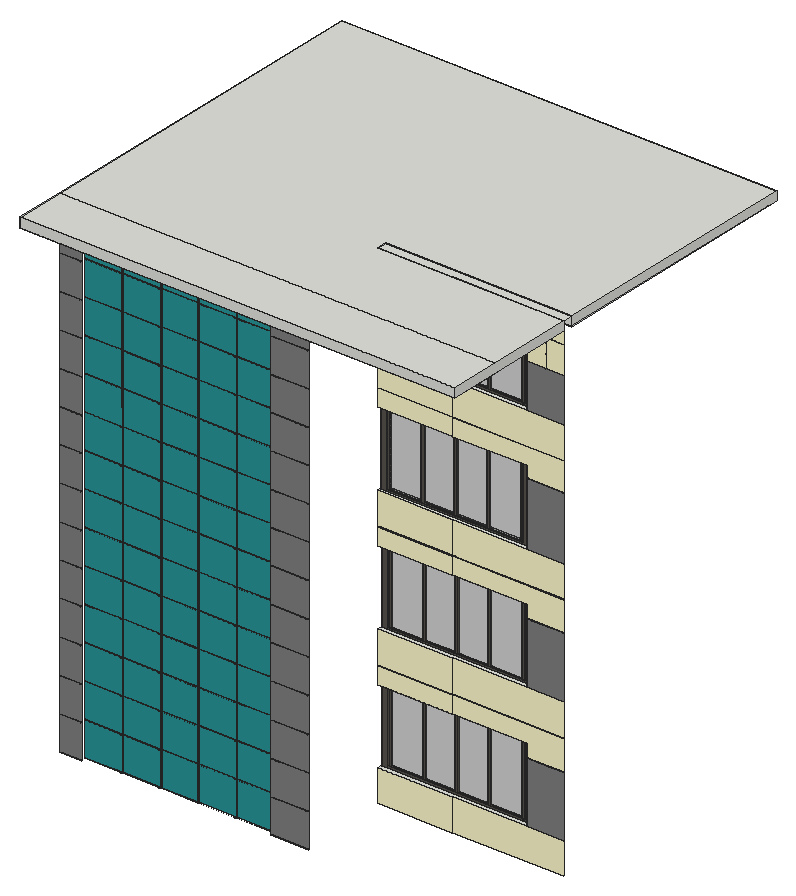
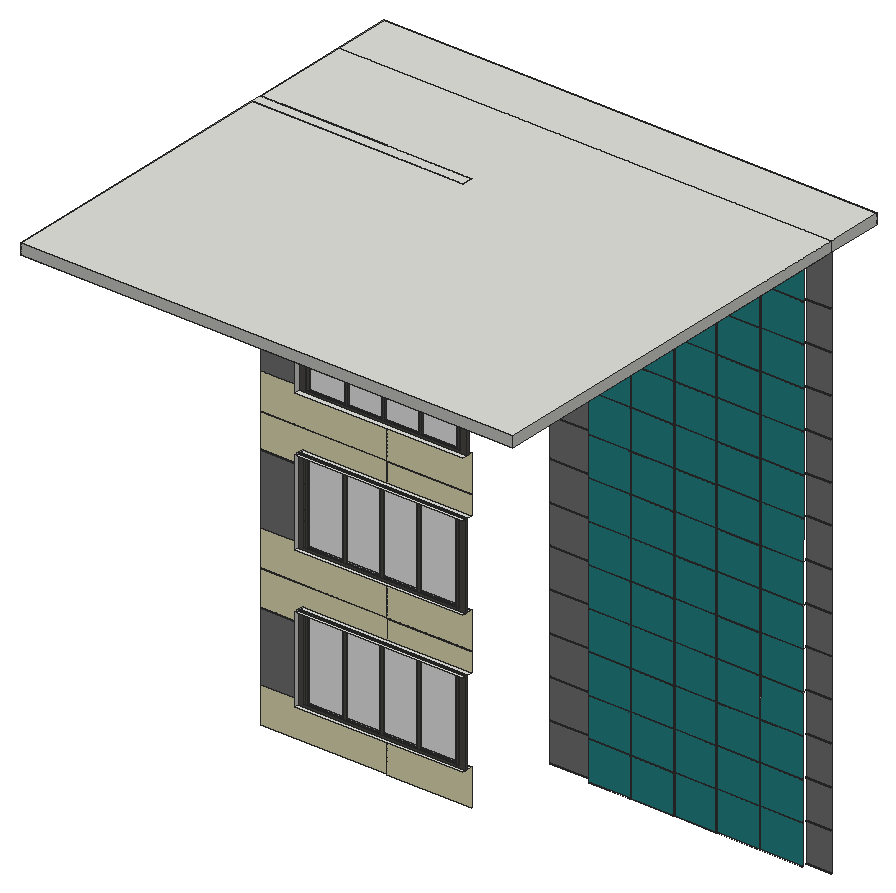
# SketchUp Ruby script. Lengths in inches.
U = 1.inch
M = Sketchup.active_model
def pt(a) = Geom::Point3d.new(a.map { |v| v * U })
def face(e, loops, mat)
  f = e.add_face(loops[0].map { |a| pt(a) })
  loops[1..].each { |l| e.add_face(l.map { |a| pt(a) }).erase! }
  f.material = f.back_material = mat if mat
  f
end
# faces: each face lists its corners as indices into pts; further lists are holes
def faces(e, pts, list, mat = nil) = list.each { |f| face(e, (f[0].is_a?(Array) ? f : [f]).map { |l| l.map { |i| pts[i] } }, mat) }
# xy, xz, yz: faces in a plane at the given z, y or x. An outline is a flat list of corners, or four numbers for a rectangle; further outlines are holes
def ring(l) = l.size == 4 ? [[l[0], l[1]], [l[2], l[1]], [l[2], l[3]], [l[0], l[3]]] : l.each_slice(2).to_a
def flat(e, list, mat, &to3) = list.each { |f| face(e, (f[0].is_a?(Array) ? f : [f]).map { |l| ring(l).map { |u, v| to3.(u, v) } }, mat) }
def xy(e, z, list, mat = nil) = flat(e, list, mat) { |x, y| [x, y, z] }
def xz(e, y, list, mat = nil) = flat(e, list, mat) { |x, z| [x, y, z] }
def yz(e, x, list, mat = nil) = flat(e, list, mat) { |y, z| [x, y, z] }
def lines(e, pts, list) = list.each { |a, b| e.add_line(pt(pts[a]), pt(pts[b])) }
# prism: a flat outline (further loops are holes) pulled along v
def prism(e, loops, v, mat = nil)
  f = face(e, loops, mat); d = Geom::Vector3d.new(v.map { |x| x * U })
  f.pushpull(f.normal.samedirection?(d) ? d.length : -d.length)
end
def box(e, o, s, mat = nil) = prism(e, [[o, [o[0] + s[0], o[1], o[2]], [o[0] + s[0], o[1] + s[1], o[2]], [o[0], o[1] + s[1], o[2]]]], [0, 0, s[2]], mat)
def at(x, y, z, deg = 0) = Geom::Transformation.translation(pt([x, y, z])) * Geom::Transformation.rotation(ORIGIN, Z_AXIS, deg.degrees)
def axes(o, x, y, z) = Geom::Transformation.new([*x, 0, *y, 0, *z, 0, *pt(o).to_a, 1])
def part(name) = M.definitions.add(name)
# library, detail: a bought-in or finely detailed component or shape, given as its bounding box
def library(name, o, s) = part(name).tap { |d| box(d.entities, o, s) }
def detail(e, o, s) = box(e.add_group.entities, o, s)
def put(e, d, t, mat = nil) = e.add_instance(d, t).tap { |i| i.material = mat if mat }
def group(e, t, mat = nil) = e.add_group.tap { |g| g.transformation = t; g.material = mat if mat }.entities
root = M.entities
M.materials.add("Aluminum_Anodized_DarkGray").color = [87, 83, 78]
M.materials.add("Glass_Coated_Black").color = [65, 65, 65]
M.materials["Glass_Coated_Black"].alpha = 0.42
M.materials.add("[0050_LemonChiffon]").color = [255, 250, 205]
M.materials.add("[0081_CadetBlue]").color = [40, 149, 153]
M.materials.add("[0133_Gray]").color = [128, 128, 128]
M.materials.add("[0137_Black]").color = [0, 0, 0]
c1 = part("Group\#2")
xy(c1.entities,0,[[0,0,54,3]],"Aluminum_Anodized_DarkGray")
xy(c1.entities,2,[[2.25,0,51.75,1],[2.25,2,51.75,3]],"Aluminum_Anodized_DarkGray")
xy(c1.entities,3,[[3.375,1,14.625,1.5],[15.75,1,26.4375,1.5],[27.5625,1,38.25,1.5],[39.375,1,50.625,1.5],[3.375,1.5,14.625,2],
  [15.75,1.5,26.4375,2],[27.5625,1.5,38.25,2],[39.375,1.5,50.625,2]],"Aluminum_Anodized_DarkGray")
xy(c1.entities,99,[[3.375,1,14.625,1.5],[15.75,1,26.4375,1.5],[26.4375,1,27.5625,2],[27.5625,1,38.25,1.5],[38.25,1,39.375,2],
  [39.375,1,50.625,1.5],[3.375,1.5,14.625,2],[15.75,1.5,26.4375,2],[27.5625,1.5,38.25,2],[39.375,1.5,50.625,2]],"Aluminum_Anodized_DarkGray")
xy(c1.entities,100,[[2.25,0,51.75,1],[2.25,2,51.75,3]],"Aluminum_Anodized_DarkGray")
xy(c1.entities,102,[[0,0,54,3]],"Aluminum_Anodized_DarkGray")
xz(c1.entities,0,[[[0,0,54,102],[2.25,2,51.75,100]]],"Aluminum_Anodized_DarkGray")
xz(c1.entities,1,[[[2.25,2,51.75,100],[39.375,3,50.625,99],[3.375,3,14.625,99],[27.5625,3,38.25,99],[15.75,3,26.4375,99]]],"Aluminum_Anodized_DarkGray")
xz(c1.entities,1.5,[[3.375,3,14.625,99],[15.75,3,27,99],[27.5625,3,38.8125,99],[39.375,3,50.625,99]],"Glass_Coated_Black")
xz(c1.entities,2,[[[2.25,2,51.75,100],[39.375,3,50.625,99],[3.375,3,14.625,99],[27.5625,3,38.25,99],[15.75,3,26.4375,99]]],"Aluminum_Anodized_DarkGray")
xz(c1.entities,3,[[[0,0,54,102],[2.25,2,51.75,100]]],"Aluminum_Anodized_DarkGray")
yz(c1.entities,0,[[0,0,3,102]],"Aluminum_Anodized_DarkGray")
yz(c1.entities,2.25,[[0,2,1,100],[2,2,3,100]],"Aluminum_Anodized_DarkGray")
yz(c1.entities,3.375,[[1,3,1.5,99],[1.5,3,2,99]],"Aluminum_Anodized_DarkGray")
yz(c1.entities,14.625,[[1,3,1.5,99],[1.5,3,2,99]],"Aluminum_Anodized_DarkGray")
yz(c1.entities,15.75,[[1,3,1.5,99],[1.5,3,2,99]],"Aluminum_Anodized_DarkGray")
yz(c1.entities,26.4375,[[1,3,2,99]],"Aluminum_Anodized_DarkGray")
yz(c1.entities,27.5625,[[1,3,1.5,99],[1.5,3,2,99]],"Aluminum_Anodized_DarkGray")
yz(c1.entities,38.25,[[1,3,2,99]],"Aluminum_Anodized_DarkGray")
yz(c1.entities,39.375,[[1,3,1.5,99],[1.5,3,2,99]],"Aluminum_Anodized_DarkGray")
yz(c1.entities,50.625,[[1,3,1.5,99],[1.5,3,2,99]],"Aluminum_Anodized_DarkGray")
yz(c1.entities,51.75,[[0,2,1,100],[2,2,3,100]],"Aluminum_Anodized_DarkGray")
yz(c1.entities,54,[[0,0,3,102]],"Aluminum_Anodized_DarkGray")
p = [[15.75,2,99],[14.625,2,99]]
lines(c1.entities,p,[[0,1]])
xy(root,530.14,[[115.9375,221.1875,136.9375,221.6875],[319.9375,221.1875,355.9375,221.75],[136.52,225.49,173.04,225.6875],[173.0625,225.49,210.01,225.6875],[210.51,225.49,246.05,225.6875],
  [246.55,225.49,283.09,225.6875],[283.59,225.49,319.625,225.6875]])
xy(root,530.64,[[115.9375,221.1875,136.9375,221.6875],[319.9375,221.1875,355.9375,221.75],[136.52,225.49,173.04,225.6875],[173.0625,225.49,210.01,225.6875],[210.51,225.49,246.05,225.6875],
  [246.55,225.49,283.09,225.6875],[283.59,225.49,319.625,225.6875]])
xy(root,562.88,[[115.9375,221.1875,136.9375,221.6875],[319.9375,221.1875,355.9375,221.6875]])
xy(root,563.38,[[115.9375,221.1875,136.9375,221.6875],[319.9375,221.1875,355.9375,221.6875],[136.49,225.49,173.03,225.6875],[173.04,225.49,210.01,225.6875],[210.51,225.49,246.05,225.6875],
  [246.55,225.49,283.09,225.6875],[283.59,225.49,319.625,225.6875]])
xy(root,563.88,[[136.49,225.49,173.02,225.6875],[173.04,225.49,210.01,225.6875],[210.51,225.49,246.05,225.6875],[246.55,225.49,283.09,225.6875],[283.59,225.49,319.625,225.6875]])
xy(root,564,[[355.9375,305.1875,499.37,314.1875]])
xy(root,596.12,[[115.9375,221.1875,136.9375,221.6875],[319.9375,221.1875,355.9375,221.6875]])
xy(root,596.62,[[115.9375,221.1875,136.9375,221.6875],[319.9375,221.1875,355.9375,221.6875],[136.45,225.49,172.99,225.6875],[173.04,225.49,210.01,225.6875],[210.51,225.49,246.05,225.6875],
  [246.55,225.49,283.09,225.6875],[283.59,225.49,319.625,225.6875]])
xy(root,597.12,[[136.45,225.49,172.99,225.6875],[173.04,225.49,210.01,225.6875],[210.51,225.49,246.05,225.6875],[246.55,225.49,283.09,225.6875],[283.59,225.49,319.625,225.6875]])
xy(root,629.36,[[115.9375,221.1875,136.9375,221.6875],[319.9375,221.1875,355.9375,221.6875]])
xy(root,629.86,[[115.9375,221.1875,136.9375,221.6875],[319.9375,221.1875,355.9375,221.6875],[136.41,225.49,172.95,225.6875],[173.04,225.49,210.01,225.6875],[210.51,225.49,246.05,225.6875],
  [246.55,225.49,283.09,225.6875],[283.59,225.49,319.625,225.6875]])
xy(root,630.36,[[136.41,225.49,172.95,225.6875],[173.04,225.49,210.01,225.6875],[210.51,225.49,246.05,225.6875],[246.55,225.49,283.09,225.6875],[283.59,225.49,319.625,225.6875]])
xy(root,636,[[355.9375,305.1875,499.37,314.1875]])
xy(root,663.1,[[115.9375,221.1875,136.9375,221.6875],[319.9375,221.1875,355.9375,221.6875],[136.375,225.49,172.91,225.6875],[173.04,225.49,210.01,225.6875],[210.51,225.49,246.05,225.6875],
  [246.55,225.49,283.09,225.6875],[283.59,225.49,319.625,225.6875]])
xy(root,663.6,[[115.9375,221.1875,136.9375,221.6875],[319.9375,221.1875,355.9375,221.6875],[136.375,225.49,172.91,225.6875],[173.04,225.49,210.01,225.6875],[210.51,225.49,246.05,225.6875],
  [246.55,225.49,283.09,225.6875],[283.59,225.49,319.625,225.6875]])
xy(root,684,[[355.9375,305.1875,499.37,314.1875]])
xy(root,696.34,[[115.9375,221.1875,136.9375,221.6875],[319.9375,221.1875,355.9375,221.6875],[136.34,225.49,172.875,225.6875],[173.04,225.49,210.01,225.6875],[210.51,225.49,246.05,225.6875],
  [246.55,225.49,283.09,225.6875],[283.59,225.49,319.625,225.6875]])
xy(root,696.84,[[115.9375,221.1875,136.9375,221.6875],[319.9375,221.1875,355.9375,221.6875],[136.34,225.49,172.875,225.6875],[173.04,225.49,210.01,225.6875],[210.51,225.49,246.05,225.6875],
  [246.55,225.49,283.09,225.6875],[283.59,225.49,319.625,225.6875]])
xy(root,729.08,[[115.9375,221.1875,136.9375,221.6875],[319.9375,221.1875,355.9375,221.6875]])
xy(root,729.58,[[115.9375,221.1875,136.9375,221.6875],[319.9375,221.1875,355.9375,221.6875],[136.3,225.49,172.84,225.6875],[173.04,225.49,210.01,225.6875],[210.51,225.49,246.05,225.6875],
  [246.55,225.49,283.09,225.6875],[283.59,225.49,319.625,225.6875]])
xy(root,730.08,[[136.3,225.49,172.84,225.6875],[173.04,225.49,210.01,225.6875],[210.51,225.49,246.05,225.6875],[246.55,225.49,283.09,225.6875],[283.59,225.49,319.625,225.6875]])
xy(root,756,[[355.9375,305.1875,499.37,314.1875]])
xy(root,762.82,[[115.9375,221.1875,136.9375,221.6875],[319.9375,221.1875,355.9375,221.6875],[136.26,225.49,172.8,225.6875],[173.04,225.49,210.01,225.6875],[210.51,225.49,246.05,225.6875],
  [246.55,225.49,283.09,225.6875],[283.59,225.49,319.625,225.6875]])
xy(root,763.32,[[115.9375,221.1875,136.9375,221.6875],[319.9375,221.1875,355.9375,221.6875],[136.26,225.49,172.8,225.6875],[173.04,225.49,210.01,225.6875],[210.51,225.49,246.05,225.6875],
  [246.55,225.49,283.09,225.6875],[283.59,225.49,319.625,225.6875]])
xy(root,796.04,[[115.9375,221.1875,136.9375,221.6875]])
xy(root,796.06,[[319.9375,221.1875,355.9375,221.6875],[136.23,225.49,172.76,225.6875],[173.04,225.49,210.01,225.6875],[210.51,225.49,246.05,225.6875],[246.55,225.49,283.09,225.6875],
  [283.59,225.49,319.625,225.6875]])
xy(root,796.56,[[115.9375,221.1875,136.9375,221.6875],[319.9375,221.1875,355.9375,221.6875],[136.23,225.49,172.76,225.6875],[173.04,225.49,210.01,225.6875],[210.51,225.49,246.05,225.6875],
  [246.55,225.49,283.09,225.6875],[283.59,225.49,319.625,225.6875]])
xy(root,804,[[355.9375,305.1875,499.37,314.1875]])
xy(root,828.8,[[115.9375,221.1875,136.9375,221.6875],[319.9375,221.1875,355.9375,221.6875]])
xy(root,829.3,[[115.9375,221.1875,136.9375,221.6875],[319.9375,221.1875,355.9375,221.6875],[136.1875,225.49,172.73,225.6875],[173.04,225.49,210.01,225.6875],[210.51,225.49,246.05,225.6875],
  [246.55,225.49,283.09,225.6875],[283.59,225.49,319.625,225.6875]])
xy(root,829.8,[[136.1875,225.49,172.73,225.6875],[173.04,225.49,210.01,225.6875],[210.51,225.49,246.05,225.6875],[246.55,225.49,283.09,225.6875],[283.59,225.49,319.625,225.6875]])
xy(root,862.04,[[115.9375,221.1875,136.9375,221.6875],[319.9375,221.1875,355.9375,221.6875]])
xy(root,862.54,[[115.9375,221.1875,136.9375,221.6875],[319.9375,221.1875,355.9375,221.6875],[136.15,225.49,172.6875,225.6875],[173.04,225.49,210.01,225.6875],[210.51,225.49,246.05,225.6875],
  [246.55,225.49,283.09,225.6875],[283.59,225.49,319.625,225.6875]])
xy(root,863.04,[[136.15,225.49,172.6875,225.6875],[173.04,225.49,210.01,225.6875],[210.51,225.49,246.05,225.6875],[246.55,225.49,283.09,225.6875],[283.59,225.49,319.625,225.6875]])
xy(root,876,[[355.9375,305.1875,499.37,314.1875]])
xy(root,895.28,[[115.9375,221.1875,136.9375,221.6875],[319.9375,221.1875,355.9375,221.6875]])
xy(root,895.78,[[115.9375,221.1875,136.9375,221.6875],[319.9375,221.1875,355.9375,221.6875],[136.11,225.49,172.65,225.6875],[173.04,225.49,210.01,225.6875],[210.51,225.49,246.05,225.6875],
  [246.55,225.49,283.09,225.6875],[283.59,225.49,319.625,225.6875]])
xy(root,896.28,[[136.11,225.49,172.65,225.6875],[173.04,225.49,210.01,225.6875],[210.51,225.49,246.05,225.6875],[246.55,225.49,283.09,225.6875],[283.59,225.49,319.625,225.6875]])
xy(root,924,[[355.9375,305.1875,499.37,314.1875]])
xy(root,928.52,[[115.9375,221.1875,136.9375,221.6875],[319.9375,221.1875,355.9375,221.6875]])
xy(root,929.02,[[115.9375,221.1875,136.9375,221.6875],[319.9375,221.1875,355.9375,221.6875],[136.08,225.49,172.61,225.6875],[173.04,225.49,210.01,225.6875],[210.51,225.49,246.05,225.6875],
  [246.55,225.49,283.09,225.6875],[283.59,225.49,319.625,225.6875]])
xy(root,929.52,[[136.08,225.49,172.61,225.6875],[173.04,225.49,210.01,225.6875],[210.51,225.49,246.05,225.6875],[246.55,225.49,283.09,225.6875],[283.59,225.49,319.625,225.6875]])
xy(root,961.76,[[115.9375,221.1875,136.9375,221.6875],[319.9375,221.1875,355.9375,221.6875]])
xy(root,962.26,[[115.9375,221.1875,136.9375,221.6875],[319.9375,221.1875,355.9375,221.6875],[136.04,225.49,172.58,225.6875],[173.04,225.49,210.01,225.6875],[210.51,225.49,246.05,225.6875],
  [246.55,225.49,283.09,225.6875],[283.59,225.49,319.625,225.6875]])
xy(root,962.76,[[136.04,225.49,172.58,225.6875],[173.04,225.49,210.01,225.6875],[210.51,225.49,246.05,225.6875],[246.55,225.49,283.09,225.6875],[283.59,225.49,319.625,225.6875]])
xy(root,981,[[355.9375,305.1875,499.37,314.1875]])
xy(root,996,[[136.9375,221.1875,319.75,230.1875],[172.54,225.49,173.04,225.6875],[210.01,225.49,210.51,225.6875],[246.05,225.49,246.55,225.6875],[283.09,225.49,283.59,225.6875]])
xy(root,1005,[[115.9375,173.1875,319.75,221.1875],[319.75,173.1875,319.9375,221.1875],[319.9375,173.1875,535.9375,221.1875],[115.9375,221.1875,319.75,230.1875],[319.75,221.1875,319.9375,552.3125],
  [319.9375,221.1875,355.9375,230.1875],[355.9375,221.1875,535.9375,230.1875],[115.9375,230.1875,115.9375,561.3125,319.75,561.3125,319.75,552.3125,124.9375,552.3125,124.9375,230.1875],[124.9375,230.1875,319.75,552.3125],[319.9375,230.1875,346.9375,552.3125],
  [346.9375,230.1875,346.9375,552.3125,319.9375,552.3125,319.9375,561.3125,355.9375,561.3125,355.9375,230.1875],[355.9375,230.1875,535.9375,305.1875],[355.9375,314.1875,535.9375,552.3125],[319.75,552.3125,319.9375,561.3125]])
xy(root,1005.1875,[[526.9375,314.1875,535.9375,552.3125],[355.9375,552.3125,535.9375,561.3125]])
xy(root,1014,[[115.9375,173.1875,535.9375,221.1875],[115.9375,221.1875,535.9375,221.1875,535.9375,305.1875,355.9375,305.1875,355.9375,314.1875,535.9375,314.1875,535.9375,561.3125,115.9375,561.3125],[355.9375,305.1875,535.9375,314.1875]])
xz(root,173.1875,[[115.9375,1005,535.9375,1014]])
xz(root,221.1875,[[319.75,996,319.9375,1005]])
xz(root,221.1875,[[115.9375,530.64,136.9375,562.88],[319.9375,530.64,355.9375,562.88],[115.9375,563.38,136.9375,596.12],[319.9375,563.38,355.9375,596.12],[115.9375,596.62,136.9375,629.36],
  [319.9375,596.62,355.9375,629.36],[115.9375,629.86,136.9375,663.1],[319.9375,629.86,355.9375,663.1],[115.9375,663.6,136.9375,696.34],[319.9375,663.6,355.9375,696.34],
  [115.9375,696.84,136.9375,729.08],[319.9375,696.84,355.9375,729.08],[115.9375,729.58,136.9375,762.82],[319.9375,729.58,355.9375,762.82],[115.9375,763.32,136.9375,796.04],
  [319.9375,763.32,355.9375,796.06],[115.9375,796.56,136.9375,828.8],[319.9375,796.56,355.9375,828.8],[115.9375,829.3,136.9375,862.04],[319.9375,829.3,355.9375,862.04],
  [115.9375,862.54,136.9375,895.28],[319.9375,862.54,355.9375,895.28],[115.9375,895.78,136.9375,928.52],[319.9375,895.78,355.9375,928.52],[115.9375,929.02,136.9375,961.76],
  [319.9375,929.02,355.9375,961.76],[115.9375,962.26,136.9375,962.26,136.9375,996,319.75,996,319.75,1005,115.9375,1005],[319.9375,962.26,355.9375,1005]],"[0133_Gray]")
xz(root,221.6875,[[115.9375,530.14,136.9375,530.64],[115.9375,562.88,136.9375,563.38],[319.9375,562.88,355.9375,563.38],[115.9375,596.12,136.9375,596.62],[319.9375,596.12,355.9375,596.62],
  [115.9375,629.36,136.9375,629.86],[319.9375,629.36,355.9375,629.86],[115.9375,663.1,136.9375,663.6],[319.9375,663.1,355.9375,663.6],[115.9375,696.34,136.9375,696.84],
  [319.9375,696.34,355.9375,696.84],[115.9375,729.08,136.9375,729.58],[319.9375,729.08,355.9375,729.58],[115.9375,762.82,136.9375,763.32],[319.9375,762.82,355.9375,763.32],
  [115.9375,796.04,136.9375,796.56],[319.9375,796.06,355.9375,796.56],[115.9375,828.8,136.9375,829.3],[319.9375,828.8,355.9375,829.3],[115.9375,862.04,136.9375,862.54],
  [319.9375,862.04,355.9375,862.54],[115.9375,895.28,136.9375,895.78],[319.9375,895.28,355.9375,895.78],[115.9375,928.52,136.9375,929.02],[319.9375,928.52,355.9375,929.02],
  [115.9375,961.76,136.9375,962.26],[319.9375,961.76,355.9375,962.26]])
xz(root,221.75,[[319.9375,530.14,355.9375,530.64]])
xz(root,225.6875,[[136.52,530.64,173.04,530.64,173.04,552.8,173.03,563.38,136.49,563.38],[173.0625,530.64,210.01,530.64,210.01,563.38,173.04,563.38,173.04,552.8],[210.51,530.64,246.05,563.38],[246.55,530.64,283.09,563.38],[283.59,530.64,319.625,563.38],
  [136.49,563.88,173.02,563.88,172.99,596.62,136.45,596.62],[173.04,563.88,210.01,596.62],[210.51,563.88,246.05,596.62],[246.55,563.88,283.09,596.62],[283.59,563.88,319.625,596.62],
  [136.45,597.12,172.99,597.12,172.95,629.86,136.41,629.86],[173.04,597.12,210.01,629.86],[210.51,597.12,246.05,629.86],[246.55,597.12,283.09,629.86],[283.59,597.12,319.625,629.86],
  [136.41,630.36,172.95,630.36,172.91,663.1,136.375,663.1],[173.04,630.36,210.01,663.1],[210.51,630.36,246.05,663.1],[246.55,630.36,283.09,663.1],[283.59,630.36,319.625,663.1],
  [136.375,663.6,172.91,663.6,172.875,696.34,136.34,696.34],[173.04,663.6,210.01,696.34],[210.51,663.6,246.05,696.34],[246.55,663.6,283.09,696.34],[283.59,663.6,319.625,696.34],
  [136.34,696.84,172.875,696.84,172.84,729.58,136.3,729.58],[173.04,696.84,210.01,729.58],[210.51,696.84,246.05,729.58],[246.55,696.84,283.09,729.58],[283.59,696.84,319.625,729.58],
  [136.3,730.08,172.84,730.08,172.8,762.82,136.26,762.82],[173.04,730.08,210.01,762.82],[210.51,730.08,246.05,762.82],[246.55,730.08,283.09,762.82],[283.59,730.08,319.625,762.82],
  [136.26,763.32,172.8,763.32,172.76,796.06,136.23,796.06],[173.04,763.32,210.01,796.06],[210.51,763.32,246.05,796.06],[246.55,763.32,283.09,796.06],[283.59,763.32,319.625,796.06],
  [136.23,796.56,172.76,796.56,172.73,829.3,136.1875,829.3],[173.04,796.56,210.01,829.3],[210.51,796.56,246.05,829.3],[246.55,796.56,283.09,829.3],[283.59,796.56,319.625,829.3],
  [136.1875,829.8,172.73,829.8,172.6875,862.54,136.15,862.54],[173.04,829.8,210.01,862.54],[210.51,829.8,246.05,862.54],[246.55,829.8,283.09,862.54],[283.59,829.8,319.625,862.54],
  [136.15,863.04,172.6875,863.04,172.65,895.78,136.11,895.78],[173.04,863.04,210.01,895.78],[210.51,863.04,246.05,895.78],[246.55,863.04,283.09,895.78],[283.59,863.04,319.625,895.78],
  [136.11,896.28,172.65,896.28,172.61,929.02,136.08,929.02],[173.04,896.28,210.01,929.02],[210.51,896.28,246.05,929.02],[246.55,896.28,283.09,929.02],[283.59,896.28,319.625,929.02],
  [136.08,929.52,172.61,929.52,172.58,962.26,136.04,962.26],[173.04,929.52,210.01,962.26],[210.51,929.52,246.05,962.26],[246.55,929.52,283.09,962.26],[283.59,929.52,319.625,962.26],
  [136.04,962.76,172.58,962.76,172.54,996,136,996],[173.04,962.76,210.01,996],[210.51,962.76,246.05,996],[246.55,962.76,283.09,996],[283.59,962.76,319.625,996]],"[0081_CadetBlue]")
xz(root,305.1875,[[499.37,622.64,535.9375,623.14],[499.37,743.48,535.9375,743.98],[499.37,864.94,535.9375,865.44],[355.9375,1005,427.65,1014],[427.65,1005,428.15,1014],
  [428.15,1005,517.9375,1014],[517.9375,1005,518.4375,1014],[518.4375,1005,535.9375,1014]])
xz(root,305.1875,[[355.9375,533.13,427.65,564],[428.15,533.13,535.9375,564],[499.37,623.14,535.9375,623.14,535.9375,652.5,428.15,652.5,428.15,636,499.37,636],[355.9375,636,427.65,652.5],[355.9375,653,427.65,684],
  [428.15,653,535.9375,684],[499.37,743.98,535.9375,743.98,535.9375,772.5,428.15,772.5,428.15,756,499.37,756],[355.9375,756,427.65,772.5],[355.9375,773,427.65,804],[428.15,773,535.9375,804],
  [499.37,865.44,535.9375,865.44,535.9375,892.5,428.15,892.5,428.15,876,499.37,876],[355.9375,876,427.65,892.5],[355.9375,893,427.65,924],[428.15,893,535.9375,924],[499.37,966.1,517.9375,966.1,517.9375,993,428.15,993,428.15,981,499.37,981],
  [518.4375,966.1,535.9375,993],[355.9375,981,427.65,993],[355.9375,993.5,427.65,1005],[428.15,993.5,517.9375,1005],[518.4375,993.5,535.9375,1005]],"[0050_LemonChiffon]")
xz(root,305.1875,[[499.37,564,535.9375,622.64],[499.37,684,535.9375,743.48],[499.37,804,535.9375,864.94],[499.37,924,535.9375,966.1]],"[0133_Gray]")
xz(root,305.1875,[[427.65,636,428.15,636,428.15,652.5,535.9375,652.5,535.9375,653,428.15,653,428.15,684,427.65,684,427.65,653,355.9375,653,355.9375,652.5,427.65,652.5],[427.65,756,428.15,772.5],[355.9375,772.5,427.65,773],[427.65,772.5,428.15,773],[428.15,772.5,535.9375,773],
  [427.65,773,428.15,804],[427.65,876,428.15,876,428.15,892.5,535.9375,892.5,535.9375,893,428.15,893,428.15,924,427.65,924,427.65,893,355.9375,893,355.9375,892.5,427.65,892.5],[517.9375,966.1,518.4375,966.1,518.4375,993,535.9375,993,535.9375,993.5,518.4375,993.5,518.4375,1005,517.9375,1005,517.9375,993.5,428.15,993.5,428.15,1005,427.65,1005,427.65,993.5,355.9375,993.5,355.9375,993,427.65,993,427.65,981,428.15,981,428.15,993,517.9375,993]],"[0137_Black]")
xz(root,314.1875,[[355.9375,1005,355.9375,1014,535.9375,1014,535.9375,1005.1875,526.9375,1005.1875,526.9375,1005],[526.9375,1005,535.9375,1005.1875]])
xz(root,552.3125,[[355.9375,1005,526.9375,1005.1875],[526.9375,1005,535.9375,1005.1875]])
xz(root,561.3125,[[115.9375,1005,115.9375,1014,535.9375,1014,535.9375,1005.1875,355.9375,1005.1875,355.9375,1005]])
yz(root,115.9375,[[173.1875,1005,221.1875,1014],[221.1875,1005,561.3125,1014]])
yz(root,136.04,[[225.49,962.26,225.6875,962.76]])
yz(root,136.08,[[225.49,929.02,225.6875,929.52]])
yz(root,136.11,[[225.49,895.78,225.6875,896.28]])
yz(root,136.15,[[225.49,862.54,225.6875,863.04]])
yz(root,136.1875,[[225.49,829.3,225.6875,829.8]])
yz(root,136.23,[[225.49,796.06,225.6875,796.56]])
yz(root,136.26,[[225.49,762.82,225.6875,763.32]])
yz(root,136.3,[[225.49,729.58,225.6875,730.08]])
yz(root,136.34,[[225.49,696.34,225.6875,696.84]])
yz(root,136.375,[[225.49,663.1,225.6875,663.6]])
yz(root,136.41,[[225.49,629.86,225.6875,630.36]])
yz(root,136.45,[[225.49,596.62,225.6875,597.12]])
yz(root,136.49,[[225.49,563.38,225.6875,563.88]])
yz(root,136.52,[[225.49,530.14,225.6875,530.64]])
yz(root,173.04,[[225.49,530.64,225.6875,552.8],[225.49,552.8,225.6875,563.38],[225.49,563.88,225.6875,596.62],[225.49,597.12,225.6875,629.86],[225.49,630.36,225.6875,663.1],
  [225.49,663.6,225.6875,696.34],[225.49,696.84,225.6875,729.58],[225.49,730.08,225.6875,762.82],[225.49,763.32,225.6875,796.06],[225.49,796.56,225.6875,829.3],
  [225.49,829.8,225.6875,862.54],[225.49,863.04,225.6875,895.78],[225.49,896.28,225.6875,929.02],[225.49,929.52,225.6875,962.26],[225.49,962.76,225.6875,996]])
yz(root,210.01,[[225.49,530.64,225.6875,563.38],[225.49,563.88,225.6875,596.62],[225.49,597.12,225.6875,629.86],[225.49,630.36,225.6875,663.1],[225.49,663.6,225.6875,696.34],
  [225.49,696.84,225.6875,729.58],[225.49,730.08,225.6875,762.82],[225.49,763.32,225.6875,796.06],[225.49,796.56,225.6875,829.3],[225.49,829.8,225.6875,862.54],
  [225.49,863.04,225.6875,895.78],[225.49,896.28,225.6875,929.02],[225.49,929.52,225.6875,962.26],[225.49,962.76,225.6875,996]])
yz(root,210.51,[[225.49,530.64,225.6875,563.38],[225.49,563.88,225.6875,596.62],[225.49,597.12,225.6875,629.86],[225.49,630.36,225.6875,663.1],[225.49,663.6,225.6875,696.34],
  [225.49,696.84,225.6875,729.58],[225.49,730.08,225.6875,762.82],[225.49,763.32,225.6875,796.06],[225.49,796.56,225.6875,829.3],[225.49,829.8,225.6875,862.54],
  [225.49,863.04,225.6875,895.78],[225.49,896.28,225.6875,929.02],[225.49,929.52,225.6875,962.26],[225.49,962.76,225.6875,996]])
yz(root,246.05,[[225.49,530.64,225.6875,563.38],[225.49,563.88,225.6875,596.62],[225.49,597.12,225.6875,629.86],[225.49,630.36,225.6875,663.1],[225.49,663.6,225.6875,696.34],
  [225.49,696.84,225.6875,729.58],[225.49,730.08,225.6875,762.82],[225.49,763.32,225.6875,796.06],[225.49,796.56,225.6875,829.3],[225.49,829.8,225.6875,862.54],
  [225.49,863.04,225.6875,895.78],[225.49,896.28,225.6875,929.02],[225.49,929.52,225.6875,962.26],[225.49,962.76,225.6875,996]])
yz(root,246.55,[[225.49,530.64,225.6875,563.38],[225.49,563.88,225.6875,596.62],[225.49,597.12,225.6875,629.86],[225.49,630.36,225.6875,663.1],[225.49,663.6,225.6875,696.34],
  [225.49,696.84,225.6875,729.58],[225.49,730.08,225.6875,762.82],[225.49,763.32,225.6875,796.06],[225.49,796.56,225.6875,829.3],[225.49,829.8,225.6875,862.54],
  [225.49,863.04,225.6875,895.78],[225.49,896.28,225.6875,929.02],[225.49,929.52,225.6875,962.26],[225.49,962.76,225.6875,996]])
yz(root,283.09,[[225.49,530.64,225.6875,563.38],[225.49,563.88,225.6875,596.62],[225.49,597.12,225.6875,629.86],[225.49,630.36,225.6875,663.1],[225.49,663.6,225.6875,696.34],
  [225.49,696.84,225.6875,729.58],[225.49,730.08,225.6875,762.82],[225.49,763.32,225.6875,796.06],[225.49,796.56,225.6875,829.3],[225.49,829.8,225.6875,862.54],
  [225.49,863.04,225.6875,895.78],[225.49,896.28,225.6875,929.02],[225.49,929.52,225.6875,962.26],[225.49,962.76,225.6875,996]])
yz(root,283.59,[[225.49,530.64,225.6875,563.38],[225.49,563.88,225.6875,596.62],[225.49,597.12,225.6875,629.86],[225.49,630.36,225.6875,663.1],[225.49,663.6,225.6875,696.34],
  [225.49,696.84,225.6875,729.58],[225.49,730.08,225.6875,762.82],[225.49,763.32,225.6875,796.06],[225.49,796.56,225.6875,829.3],[225.49,829.8,225.6875,862.54],
  [225.49,863.04,225.6875,895.78],[225.49,896.28,225.6875,929.02],[225.49,929.52,225.6875,962.26],[225.49,962.76,225.6875,996]])
yz(root,319.625,[[225.49,530.14,225.6875,530.64],[225.49,563.38,225.6875,563.88],[225.49,596.62,225.6875,597.12],[225.49,629.86,225.6875,630.36],[225.49,663.1,225.6875,663.6],
  [225.49,696.34,225.6875,696.84],[225.49,729.58,225.6875,730.08],[225.49,762.82,225.6875,763.32],[225.49,796.06,225.6875,796.56],[225.49,829.3,225.6875,829.8],
  [225.49,862.54,225.6875,863.04],[225.49,895.78,225.6875,896.28],[225.49,929.02,225.6875,929.52],[225.49,962.26,225.6875,962.76]])
yz(root,319.75,[[221.1875,996,230.1875,1005]])
yz(root,355.9375,[[305.1875,1005,314.1875,1014],[552.3125,1005,561.3125,1005.1875]])
yz(root,499.37,[[305.1875,564,314.1875,636],[305.1875,684,314.1875,756],[305.1875,804,314.1875,876],[305.1875,924,314.1875,981]])
yz(root,535.9375,[[173.1875,1005,305.1875,1014],[314.1875,1005,552.3125,1005.1875],[314.1875,1005.1875,561.3125,1014]])
p = [[173.0625,225.6875,530.64],[173.04,225.6875,552.8],[173.04,225.49,552.8],[173.0625,225.49,530.64],[173.03,225.6875,563.38],[173.03,225.49,563.38],
  [172.99,225.6875,596.62],[173.02,225.6875,563.88],[173.02,225.49,563.88],[172.99,225.49,596.62],[172.95,225.6875,629.86],[172.99,225.6875,597.12],
  [172.99,225.49,597.12],[172.95,225.49,629.86],[172.91,225.6875,663.1],[172.95,225.6875,630.36],[172.95,225.49,630.36],[172.91,225.49,663.1],
  [172.875,225.6875,696.34],[172.91,225.6875,663.6],[172.91,225.49,663.6],[172.875,225.49,696.34],[172.84,225.6875,729.58],[172.875,225.6875,696.84],
  [172.875,225.49,696.84],[172.84,225.49,729.58],[172.8,225.6875,762.82],[172.84,225.6875,730.08],[172.84,225.49,730.08],[172.8,225.49,762.82],
  [172.76,225.6875,796.06],[172.8,225.6875,763.32],[172.8,225.49,763.32],[172.76,225.49,796.06],[172.73,225.6875,829.3],[172.76,225.6875,796.56],
  [172.76,225.49,796.56],[172.73,225.49,829.3],[172.6875,225.6875,862.54],[172.73,225.6875,829.8],[172.73,225.49,829.8],[172.6875,225.49,862.54],
  [172.65,225.6875,895.78],[172.6875,225.6875,863.04],[172.6875,225.49,863.04],[172.65,225.49,895.78],[172.61,225.6875,929.02],[172.65,225.6875,896.28],
  [172.65,225.49,896.28],[172.61,225.49,929.02],[172.58,225.6875,962.26],[172.61,225.6875,929.52],[172.61,225.49,929.52],[172.58,225.49,962.26],
  [172.54,225.6875,996],[172.58,225.6875,962.76],[172.58,225.49,962.76],[172.54,225.49,996]]
faces(root,p,[[0,1,2,3],[4,1,2,5],[6,7,8,9],[10,11,12,13],[14,15,16,17],[18,19,20,21],[22,23,24,25],[26,27,28,29],
  [30,31,32,33],[34,35,36,37],[38,39,40,41],[42,43,44,45],[46,47,48,49],[50,51,52,53],[54,55,56,57]])
put(root,c1,axes([355.9375,309.6875,564],[2.66667,0,0],[0,0.5,0],[0,0,0.71]))
put(root,c1,axes([355.9375,309.6875,684],[2.66667,0,0],[0,0.5,0],[0,0,0.71]))
put(root,c1,axes([355.9375,308.1875,804],[2.66667,0,0],[0,0.5,0],[0,0,0.71]))
put(root,c1,axes([355.9375,309.6875,924],[2.66667,0,0],[0,0.5,0],[0,0,0.71]))
